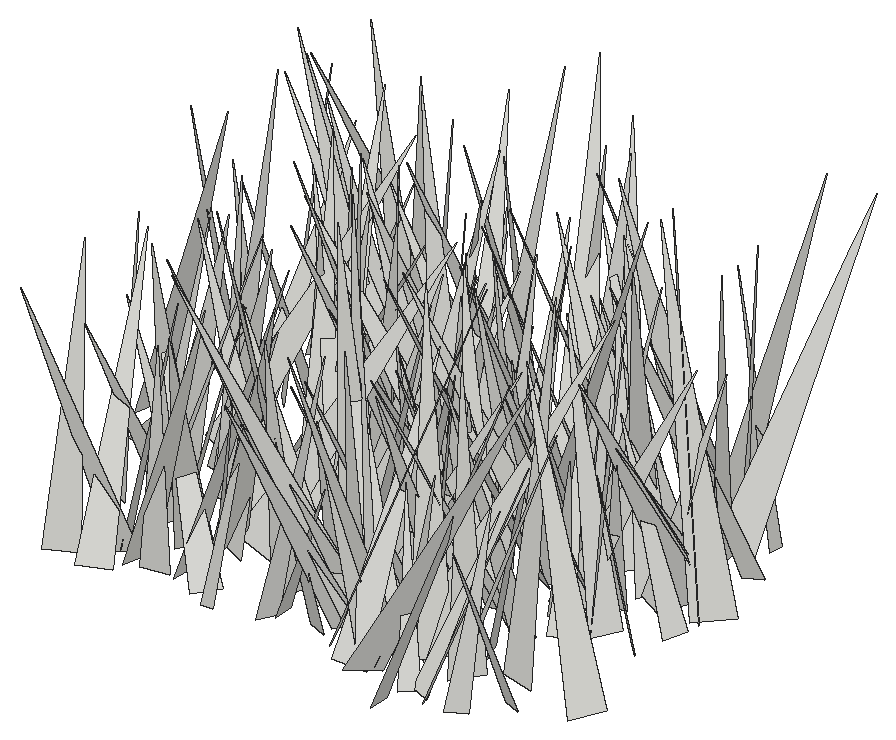
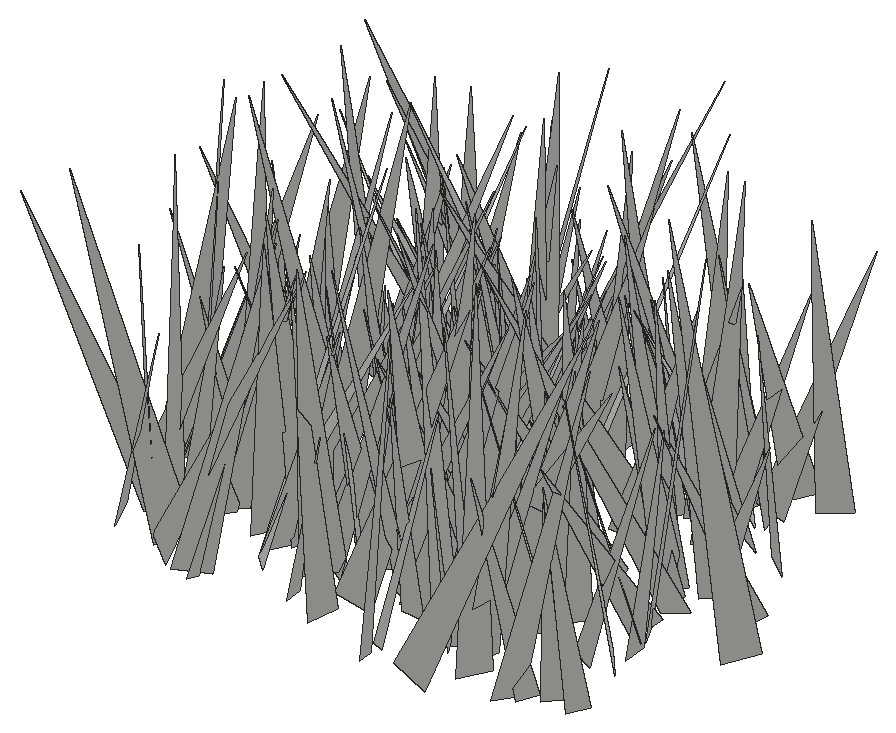
# SketchUp Ruby script. Lengths in inches.
U = 1.inch
M = Sketchup.active_model
def pt(a) = Geom::Point3d.new(a.map { |v| v * U })
def face(e, loops, mat)
  f = e.add_face(loops[0].map { |a| pt(a) })
  loops[1..].each { |l| e.add_face(l.map { |a| pt(a) }).erase! }
  f.material = f.back_material = mat if mat
  f
end
# faces: each face lists its corners as indices into pts; further lists are holes
def faces(e, pts, list, mat = nil) = list.each { |f| face(e, (f[0].is_a?(Array) ? f : [f]).map { |l| l.map { |i| pts[i] } }, mat) }
# xy, xz, yz: faces in a plane at the given z, y or x. An outline is a flat list of corners, or four numbers for a rectangle; further outlines are holes
def ring(l) = l.size == 4 ? [[l[0], l[1]], [l[2], l[1]], [l[2], l[3]], [l[0], l[3]]] : l.each_slice(2).to_a
def flat(e, list, mat, &to3) = list.each { |f| face(e, (f[0].is_a?(Array) ? f : [f]).map { |l| ring(l).map { |u, v| to3.(u, v) } }, mat) }
def xy(e, z, list, mat = nil) = flat(e, list, mat) { |x, y| [x, y, z] }
def xz(e, y, list, mat = nil) = flat(e, list, mat) { |x, z| [x, y, z] }
def yz(e, x, list, mat = nil) = flat(e, list, mat) { |y, z| [x, y, z] }
def lines(e, pts, list) = list.each { |a, b| e.add_line(pt(pts[a]), pt(pts[b])) }
# prism: a flat outline (further loops are holes) pulled along v
def prism(e, loops, v, mat = nil)
  f = face(e, loops, mat); d = Geom::Vector3d.new(v.map { |x| x * U })
  f.pushpull(f.normal.samedirection?(d) ? d.length : -d.length)
end
def box(e, o, s, mat = nil) = prism(e, [[o, [o[0] + s[0], o[1], o[2]], [o[0] + s[0], o[1] + s[1], o[2]], [o[0], o[1] + s[1], o[2]]]], [0, 0, s[2]], mat)
def at(x, y, z, deg = 0) = Geom::Transformation.translation(pt([x, y, z])) * Geom::Transformation.rotation(ORIGIN, Z_AXIS, deg.degrees)
def axes(o, x, y, z) = Geom::Transformation.new([*x, 0, *y, 0, *z, 0, *pt(o).to_a, 1])
def part(name) = M.definitions.add(name)
# library, detail: a bought-in or finely detailed component or shape, given as its bounding box
def library(name, o, s) = part(name).tap { |d| box(d.entities, o, s) }
def detail(e, o, s) = box(e.add_group.entities, o, s)
def put(e, d, t, mat = nil) = e.add_instance(d, t).tap { |i| i.material = mat if mat }
def group(e, t, mat = nil) = e.add_group.tap { |g| g.transformation = t; g.material = mat if mat }.entities
root = M.entities
c1 = part("fur_instance\#9")
p = [[0.8125,0,1.79],[0.67,-0.02,1.48],[0,-0.11,0],[0,0.11,0]]
faces(c1.entities,p,[[0,1,2,3]])
put(root,c1,axes([517.64,24.74,-21.86],[1.43774,-5.64122,0.58152],[-5.34924,-1.54822,-1.79367],[-1.88339,0.09091,5.53834]))
put(root,c1,axes([526.01,23.85,-21.86],[-1.2303,-3.6424,0.32202],[-3.65502,1.23499,0.00478],[0.10759,0.30356,3.84457]))
put(root,c1,axes([524.72,22.25,-21.86],[-2.57998,2.99071,1.64125],[3.02202,2.95835,-0.64026],[1.58287,-0.77341,3.89753]))
put(root,c1,axes([518.1875,25.03,-21.86],[-8.04638,-2.10125,0.20494],[-2.02323,7.90531,1.61682],[0.60315,-1.51404,8.15753]))
put(root,c1,axes([519.22,25.19,-21.86],[-6.19203,-3.31038,1.54754],[-2.85802,6.28451,2.00782],[2.2771,-1.114,6.72819]))
put(root,c1,axes([507.86,24.08,-21.86],[-0.4063,-5.76079,1.26429],[-5.69006,0.04941,-1.60344],[-1.5519,1.32705,5.54804]))
put(root,c1,axes([508.55,24.05,-21.86],[6.83641,-1.96558,0.32372],[-1.94381,-6.83529,-0.45298],[-0.43579,-0.34652,7.09893]))
put(root,c1,axes([509.57,23.6,-21.86],[1.49528,-4.80686,1.53266],[-5.04418,-1.45777,0.34917],[-0.10564,1.56838,5.02194]))
put(root,c1,axes([522.05,21.04,-21.86],[6.47636,2.00005,0.90058],[1.74291,-6.39683,1.67254],[-1.33173,1.35459,6.56857]))
put(root,c1,axes([519.69,23.4375,-21.86],[-4.79801,0.15244,1.14259],[0.25589,4.91001,0.4195],[1.12396,-0.46714,4.78206]))
put(root,c1,axes([520.09,22.57,-21.86],[7.15691,-3.14413,0.26361],[-3.09126,-6.8566,2.14652],[0.63178,2.06831,7.5166]))
put(root,c1,axes([505.98,22.61,-21.86],[3.27303,-4.65782,3.06275],[-5.40234,-3.52629,0.41046],[-1.37496,2.76738,5.67799]))
put(root,c1,axes([522.38,22.42,-21.86],[-3.13044,2.30171,0.23571],[2.28042,3.13636,-0.34054],[0.39127,0.13578,3.8706]))
put(root,c1,axes([515.16,24.08,-21.86],[3.6641,-0.22277,0.06955],[-0.2117,-3.63329,-0.48425],[-0.09821,-0.47926,3.63879]))
put(root,c1,axes([509.48,25.99,-21.86],[4.70982,-4.44224,0.12242],[-4.38661,-4.67586,-0.90827],[-0.71149,-0.57769,6.41023]))
put(root,c1,axes([517.25,26.03,-21.86],[3.98276,-1.20965,1.22676],[-0.42908,-3.68899,-2.24451],[-1.66855,-1.93873,3.5054]))
put(root,c1,axes([522.8125,22.5,-21.86],[0.96645,3.75371,0.08435],[3.72936,-0.9496,-0.47076],[0.43512,-0.19848,3.84744]))
put(root,c1,axes([521.02,23.74,-21.86],[4.01363,-0.60213,1.19124],[-0.70216,-4.16285,0.26162],[-1.13516,0.446,4.0501]))
put(root,c1,axes([518.45,24.46,-21.86],[5.75232,0.0292,2.58276],[0.25276,-6.28131,-0.49192],[-2.57052,-0.55229,5.73133]))
put(root,c1,axes([514.51,25.16,-21.86],[5.42089,-2.3865,1.81758],[-2.19868,-5.71457,-0.94576],[-2.04078,-0.18248,5.84696]))
put(root,c1,axes([520.23,23.57,-21.86],[5.44846,0.74036,0.07595],[0.73692,-5.44519,0.21553],[-0.10422,0.20337,5.4943]))
put(root,c1,axes([523.26,22.27,-21.86],[4.24517,2.47398,0.29086],[2.34061,-4.15824,1.20716],[-0.85248,0.90284,4.76286]))
put(root,c1,axes([516.91,23.9,-21.86],[-5.12266,-6.1706,2.10185],[-6.50165,4.64284,-2.21548],[-0.47189,3.01719,7.70776]))
put(root,c1,axes([514.92,23.48,-21.86],[5.08359,-0.28901,1.82683],[-0.68576,-5.25683,1.07667],[-1.71772,1.24337,4.97667]))
put(root,c1,axes([523.4,24.53,-21.86],[4.8811,-3.48072,2.77846],[-3.79933,-5.40519,-0.09683],[-2.32386,1.52607,5.99426]))
put(root,c1,axes([523.51,23.6,-21.86],[4.74716,3.3592,0.52437],[3.38285,-4.75689,-0.1518],[-0.33985,-0.42721,5.81349]))
put(root,c1,axes([511.97,23.61,-21.86],[-3.53792,4.34861,0.23075],[4.30519,3.44804,1.02808],[-0.65501,-0.82532,5.51093]))
put(root,c1,axes([519.49,22.55,-21.86],[-1.69129,6.09931,0.73665],[6.01995,1.79783,-1.06428],[1.22654,-0.41345,6.23934]))
put(root,c1,axes([516.08,26.26,-21.86],[4.34393,-1.36952,0.92271],[-1.07858,-4.31928,-1.3331],[-1.25046,-1.03195,4.35524]))
put(root,c1,axes([511.19,25.16,-21.86],[3.83115,1.46002,1.29175],[1.69697,-3.89964,-0.62537],[-0.95945,-1.06731,4.05194]))
put(root,c1,axes([507.37,24.68,-21.86],[5.01565,1.80166,1.23073],[1.89818,-5.12441,-0.23415],[-1.07592,-0.64182,5.32428]))
put(root,c1,axes([514.25,27.18,-21.86],[-5.96811,-4.81477,0.42538],[-4.75156,5.96808,0.88657],[0.88638,-0.42578,7.61672]))
put(root,c1,axes([507.65,22.45,-21.86],[-4.47188,4.60163,0.40246],[4.4512,4.44255,-1.33612],[1.23441,0.65071,6.27595]))
put(root,c1,axes([512.72,22.71,-21.86],[2.07794,4.44656,0.23399],[4.16362,-2.03187,1.63715],[-1.57826,0.49406,4.62704]))
put(root,c1,axes([510.54,26.67,-21.86],[6.88515,-2.28469,0.18682],[-2.24647,-6.84269,-0.88939],[-0.45618,-0.78602,7.19959]))
put(root,c1,axes([507.83,27.18,-21.86],[0.74185,-5.118,0.35857],[-5.01336,-0.80012,-1.04825],[-1.09027,0.19676,5.06413]))
put(root,c1,axes([510.47,24.18,-21.86],[6.55283,1.12937,1.12544],[0.97488,-6.60494,0.95181],[-1.26162,0.76214,6.58096]))
put(root,c1,axes([520.47,27.45,-21.86],[1.50349,-5.86365,0.5049],[-5.82358,-1.55753,-0.74685],[-0.85041,0.2992,6.00709]))
put(root,c1,axes([515.95,25.72,-21.86],[-5.32926,2.77314,1.19327],[2.9808,5.21718,1.1879],[0.47858,-1.6143,5.88899]))
put(root,c1,axes([528.59,25.03,-21.86],[-5.76808,3.66085,1.08427],[3.77252,5.76709,0.59739],[0.58783,-1.08949,6.80556]))
put(root,c1,axes([521.47,24.82,-21.86],[-5.69,4.35692,2.08043],[4.49689,5.95288,-0.16772],[1.75752,-1.1258,7.16454]))
put(root,c1,axes([508.03,27.28,-21.86],[4.78165,-4.93816,1.39024],[-4.88475,-4.96331,-0.82896],[-1.56762,0.40313,6.82367]))
put(root,c1,axes([517.77,23.82,-21.86],[6.75975,3.62956,0.52461],[3.54067,-6.74583,1.04905],[-0.95528,0.68056,7.60048]))
put(root,c1,axes([522,28.78,-21.86],[-4.86076,-4.47494,0.06756],[-4.36579,4.76306,1.38194],[0.98465,-0.972,6.46083]))
put(root,c1,axes([519.0625,25.1,-21.86],[-4.60264,5.20733,0.96805],[5.29634,4.53648,0.77902],[0.04773,-1.24166,6.90606]))
put(root,c1,axes([519.39,26.97,-21.86],[-2.08811,-4.65792,0.59921],[-4.45757,1.75934,-1.85749],[-1.47829,1.27435,4.7546]))
put(root,c1,axes([516.67,26.875,-21.86],[-4.81324,5.46383,3.73935],[6.29264,5.21276,0.48307],[2.05886,-3.15867,7.26549]))
put(root,c1,axes([518.51,24.67,-21.86],[1.43872,7.93621,2.15807],[7.82752,-1.99366,2.11323],[-2.52399,-1.65906,7.7838]))
put(root,c1,axes([525.0625,25.375,-21.86],[2.04699,7.14679,2.15899],[7.40344,-2.23185,0.36858],[-0.96272,-1.9673,7.42502]))
put(root,c1,axes([511.01,26.4,-21.86],[1.57919,4.13225,1.33364],[4.34025,-1.54395,-0.35548],[-0.12772,-1.37428,4.40942]))
put(root,c1,axes([519.71,26.97,-21.86],[4.70905,2.28139,1.77217],[2.5251,-4.89691,-0.40574],[-1.40329,-1.15586,5.21682]))
put(root,c1,axes([520.86,24.77,-21.86],[2.72489,7.5123,0.23605],[7.26372,-2.56761,-2.13568],[1.931,-0.94238,7.70056]))
put(root,c1,axes([523.02,28.23,-21.86],[-0.18696,-5.47828,1.21386],[-5.53827,-0.01495,-0.92048],[-0.90141,1.22808,5.40363]))
put(root,c1,axes([508.27,24.54,-21.86],[4.52328,4.39752,0.22155],[4.10164,-4.32376,2.0806],[-1.60118,1.34692,5.95561]))
put(root,c1,axes([515.49,29.15,-21.86],[-3.4189,-2.83051,0.24342],[-2.77437,3.40847,0.66713],[0.61145,-0.36118,4.38812]))
put(root,c1,axes([517.16,28.14,-21.86],[2.82245,-3.27125,1.23973],[-3.47956,-2.78972,0.56063],[-0.36142,1.31172,4.28404]))
put(root,c1,axes([505.17,27.0625,-21.86],[2.73063,4.59292,1.67983],[4.59916,-3.06583,0.90635],[-1.66266,-0.93747,5.2659]))
put(root,c1,axes([522.95,26.5,-21.86],[6.22186,3.72093,2.03459],[3.43335,-6.54009,1.46143],[-2.48938,0.27987,7.10078]))
put(root,c1,axes([519.5,28.74,-21.86],[-3.50463,1.38607,1.3282],[1.66931,3.56562,0.68373],[0.94799,-1.15452,3.70623]))
put(root,c1,axes([507.08,26.35,-21.86],[2.36342,5.34352,0.74133],[5.25737,-2.46286,0.99138],[-1.20944,-0.26392,5.75813]))
put(root,c1,axes([507.03,28.88,-21.86],[4.88196,1.64498,0.71636],[1.77456,-4.73338,-1.22423],[-0.26474,-1.39349,5.00407]))
put(root,c1,axes([520.94,29.14,-21.86],[-1.8038,-4.78632,0.84713],[-4.75617,1.55162,-1.36069],[-1.00264,1.25053,4.93062]))
put(root,c1,axes([523.84,31.3,-21.86],[-2.90473,-5.90083,0.221],[-5.68544,2.86131,1.67173],[1.5951,-0.54696,6.36102]))
put(root,c1,axes([517.11,27.54,-21.86],[2.90433,5.023,0.38727],[4.82562,-2.64532,-1.87916],[1.44702,-1.25991,5.48948]))
put(root,c1,axes([523.43,29.86,-21.86],[0.93641,-4.49496,0.58968],[-4.44892,-0.79539,1.00188],[0.87152,0.76939,4.48082]))
put(root,c1,axes([515.24,28.85,-21.86],[5.83146,1.27805,1.15338],[1.33487,-5.92923,-0.17895],[-1.08712,-0.42484,5.96719]))
put(root,c1,axes([510.91,28.69,-21.86],[-2.86629,5.19134,1.30889],[5.27356,2.48156,1.70596],[-0.92348,-1.94182,5.67938]))
put(root,c1,axes([520.86,31.95,-21.86],[-3.40543,-6.99905,0.02732],[-6.9991,3.40539,-0.01642],[-0.00281,0.03175,7.78353]))
put(root,c1,axes([518.53,30.54,-21.86],[-3.7934,-3.57067,0.95546],[-3.47781,3.9116,0.81037],[1.25196,0.04698,5.14615]))
put(root,c1,axes([511.25,27.2,-21.86],[-0.59602,7.49567,1.64856],[6.68012,1.32078,-3.59019],[3.77872,-1.15261,6.60687]))
put(root,c1,axes([526.86,29.875,-21.86],[-2.53419,-2.69204,0.92744],[-2.77792,2.61003,-0.01451],[0.6248,0.68554,3.69715]))
put(root,c1,axes([507.12,30.71,-21.86],[1.45023,-6.39796,1.08768],[-6.25164,-1.07813,1.99368],[1.74182,1.45734,6.24998]))
put(root,c1,axes([506.11,29.1875,-21.86],[-1.40668,3.30295,0.84871],[3.29754,1.08331,1.24951],[-0.86952,-1.23511,3.36556]))
put(root,c1,axes([521.91,32.16,-21.86],[2.52782,-6.77606,0.30453],[-6.73549,-2.54598,-0.74076],[-0.80053,0.02468,7.19418]))
put(root,c1,axes([505.4,30.24,-21.86],[2.93008,-5.46925,1.49234],[-5.65269,-2.69042,1.23848],[0.43226,1.89052,6.07982]))
put(root,c1,axes([508.35,29.22,-21.86],[1.54209,5.92638,1.72605],[6.04197,-1.81335,0.82809],[-1.2633,-1.43843,6.06748]))
put(root,c1,axes([524.21,28.9375,-21.86],[-1.31854,4.49628,0.43937],[4.51767,1.31381,0.11263],[0.01505,-0.45333,4.68427]))
put(root,c1,axes([506.58,31.32,-21.86],[1.31964,-4.20384,0.49444],[-3.9297,-1.02429,1.77946],[1.57296,0.96785,4.03079]))
put(root,c1,axes([503.22,30.69,-21.86],[2.58418,-3.37784,0.00054],[-2.92311,-2.23595,2.1316],[1.69269,1.29557,3.68023]))
put(root,c1,axes([519.58,30.18,-21.86],[-3.57367,4.96866,1.72232],[5.21894,3.60663,0.42422],[0.64547,-1.65218,6.10563]))
put(root,c1,axes([525.36,30.16,-21.86],[-5.60882,2.54428,1.1021],[2.59069,5.69507,0.03704],[0.9881,-0.48955,6.15881]))
put(root,c1,axes([524.33,31.97,-21.86],[0.84886,-4.32385,0.54485],[-4.30912,-0.7498,0.76315],[0.65118,0.6747,4.3398]))
put(root,c1,axes([524.64,30.01,-21.86],[-3.91577,-3.49387,3.17429],[-4.26524,4.38586,-0.43413],[2.02262,2.48468,5.2299]))
put(root,c1,axes([514.11,30.24,-21.86],[-0.00345,4.9845,1.60202],[5.18158,-0.22632,0.71534],[-0.75028,-1.58596,4.93291]))
put(root,c1,axes([526.41,34.08,-21.86],[4.00993,-5.51552,0.33203],[-5.14979,-3.87921,-2.24547],[-2.00271,-1.06842,6.43882]))
put(root,c1,axes([520.71,32.9375,-21.86],[-6.87561,-0.89332,0.66489],[-0.69538,6.69239,1.80069],[0.86979,-1.71115,6.69549]))
put(root,c1,axes([523.125,30.48,-21.86],[0.63179,6.0642,2.01169],[5.81387,0.29266,-2.70812],[2.6496,-2.08816,5.46258]))
put(root,c1,axes([518.3,31.92,-21.86],[-2.43401,-4.94438,0.27236],[-4.40728,2.02468,-2.63096],[-2.25763,1.37813,4.84245]))
put(root,c1,axes([517.22,32.18,-21.86],[2.03296,-3.43324,0.36978],[-3.45285,-2.01606,0.26469],[0.04074,0.45292,3.9812]))
put(root,c1,axes([522.57,32.8,-21.86],[-1.29347,-4.18784,0.40951],[-4.17089,1.33267,0.45438],[0.55623,0.25449,4.35943]))
put(root,c1,axes([515.72,31.0625,-21.86],[5.7925,1.49056,1.34896],[1.52882,-5.93778,-0.00376],[-1.30544,-0.3399,5.9812]))
put(root,c1,axes([512.96,31.46,-21.86],[-2.66914,2.15187,1.53787],[2.38339,2.90414,0.07299],[1.14676,-1.02728,3.42776]))
put(root,c1,axes([523.29,31.23,-21.86],[-2.34168,-2.41248,1.9117],[-2.76899,2.70012,0.01564],[1.3444,1.35921,3.36204]))
put(root,c1,axes([527.4,31.65,-21.86],[-3.9914,1.89648,0.82188],[2.01712,3.964,0.64912],[0.45094,-0.94526,4.3711]))
put(root,c1,axes([514.66,33.35,-21.86],[-0.7364,-6.55979,0.93298],[-6.36781,0.44127,-1.92351],[-1.83094,1.10364,6.31453]))
put(root,c1,axes([515.47,31.5,-21.86],[-1.82115,-3.36265,1.61921],[-3.73204,1.65736,-0.7556],[0.03439,1.7865,3.74875]))
put(root,c1,axes([512.54,31.41,-21.86],[4.06784,5.47307,2.7985],[5.78633,-4.54195,0.47187],[-2.07475,-1.93641,6.80288]))
put(root,c1,axes([519.1,30.01,-21.86],[-6.05954,0.33778,0.89505],[0.02694,5.79744,-2.00555],[0.95629,1.97708,5.728]))
put(root,c1,axes([501.85,33.27,-21.86],[8.0282,-2.33719,0.44231],[-2.30718,-8.02996,-0.55383],[-0.57877,-0.40914,8.34313]))
put(root,c1,axes([517.36,31.74,-21.86],[-1.86227,-3.58892,1.59018],[-3.91628,1.57852,-1.02377],[-0.26793,1.87217,3.91156]))
put(root,c1,axes([526.7,35.01,-21.86],[-4.06772,-3.26977,0.32403],[-2.78571,3.7053,2.41936],[1.74246,-1.70943,4.62433]))
put(root,c1,axes([511.43,30.99,-21.86],[1.43263,3.39143,0.32506],[3.34277,-1.46736,0.57677],[-0.65831,-0.07043,3.63615]))
put(root,c1,axes([515.86,33.27,-21.86],[4.04014,-3.74392,1.13553],[-3.80741,-4.13804,-0.09691],[-0.90002,0.69913,5.50729]))
put(root,c1,axes([505.65,33.9375,-21.86],[-6.01698,-4.0059,2.23214],[-3.85326,6.41302,1.12219],[2.48637,0.24439,7.14087]))
put(root,c1,axes([519.27,31.54,-21.86],[1.06492,5.99669,1.55027],[6.17359,-1.15473,0.22589],[-0.50038,-1.48458,6.08632]))
put(root,c1,axes([514.15,33.63,-21.86],[-5.99234,-4.15881,0.58341],[-4.19764,5.96205,-0.6148],[0.12593,0.83815,7.26814]))
put(root,c1,axes([511.26,30.85,-21.86],[-5.83364,4.02968,1.05878],[3.90844,5.92385,-1.01134],[1.44341,0.24573,7.01761]))
put(root,c1,axes([512.14,31.56,-21.86],[-5.57386,3.34507,0.61319],[3.34749,5.6042,-0.14346],[0.5998,-0.19191,6.49898]))
put(root,c1,axes([510.21,33.02,-21.86],[5.45486,-2.53583,1.72286],[-2.73109,-5.61705,0.37948],[-1.39279,1.08278,6.00349]))
put(root,c1,axes([518.63,33.77,-21.86],[0.40641,-5.35004,1.66525],[-5.54368,-0.62666,-0.66032],[-0.81458,1.59547,5.32467]))
put(root,c1,axes([507.16,30.78,-21.86],[-7.30658,0.78889,2.52937],[0.00726,7.42557,-2.29501],[2.64953,2.15518,6.98151]))
put(root,c1,axes([518.52,34.28,-21.86],[4.42301,-0.66017,1.25029],[-0.31732,-4.46498,-1.23502],[-1.37781,-1.09094,4.29808]))
put(root,c1,axes([515.54,34.4375,-21.86],[-6.69596,1.51903,0.23584],[1.52209,6.40398,1.96756],[-0.2152,-1.96993,6.57815]))
put(root,c1,axes([515.375,30.52,-21.86],[1.15921,7.66569,0.40932],[7.66684,-1.17697,0.3294],[-0.3873,-0.35503,7.74584]))
put(root,c1,axes([517.72,32.74,-21.86],[2.94995,3.39967,1.09614],[3.50655,-3.02709,-0.04841],[-0.68072,-0.86052,4.50085]))
put(root,c1,axes([508.97,31.46,-21.86],[5.85572,0.96623,0.0245],[0.91904,-5.61274,1.69591],[-0.29926,1.66948,5.68743]))
put(root,c1,axes([512.08,33.45,-21.86],[-0.77614,4.62516,2.62163],[4.88719,1.66369,-1.48826],[2.09294,-2.16967,4.44742]))
put(root,c1,axes([522.83,35.64,-21.86],[0.39282,-7.92697,1.06347],[-7.86049,-0.18606,1.51663],[1.47665,1.11832,7.79044]))
put(root,c1,axes([519.61,33.48,-21.86],[8.28106,0.30024,0.90595],[0.31898,-8.32832,-0.15571],[-0.89952,-0.18935,8.28504]))
put(root,c1,axes([525.25,32.89,-21.86],[2.00403,4.77087,1.2081],[4.88814,-1.77806,-1.08691],[0.57161,-1.52123,5.05925]))
put(root,c1,axes([508.25,34.8,-21.86],[5.02867,-2.50397,0.95955],[-2.41233,-5.11484,-0.70513],[-1.17101,-0.21602,5.57317]))
put(root,c1,axes([520.79,34.5,-21.86],[-2.94744,-5.34651,0.76174],[-5.29498,2.69026,-1.60576],[-1.06233,1.42484,5.89017]))
put(root,c1,axes([527.79,33.42,-21.86],[-4.55755,6.1935,2.40469],[6.62517,4.45559,1.08074],[0.49905,-2.58872,7.61332]))
put(root,c1,axes([527.07,33.33,-21.86],[-5.85102,-5.01294,3.05498],[-5.59861,6.06235,-0.77491],[1.76582,2.61061,7.66574]))
put(root,c1,axes([505.875,32.04,-21.86],[1.59933,7.72158,1.03232],[7.26868,-1.09996,-3.03359],[2.80263,-1.55359,7.2786]))
put(root,c1,axes([512.26,33.94,-21.86],[4.77754,4.17311,2.72058],[4.61145,-5.13068,-0.22808],[-1.8844,-1.97551,6.33938]))
put(root,c1,axes([511.39,31.11,-21.86],[-1.39232,7.88876,0.40308],[7.89477,1.37627,0.33483],[-0.26016,-0.45487,8.00369]))
put(root,c1,axes([510.87,35.13,-21.86],[0.4901,-6.09421,1.40714],[-6.12992,-0.18765,1.32232],[1.24239,1.47818,5.96918]))
put(root,c1,axes([512.84,32.0625,-21.86],[-3.36626,3.2291,1.55087],[2.48228,3.63709,-2.18492],[2.58275,0.71309,4.12128]))
put(root,c1,axes([523.21,31.53,-21.86],[3.09687,5.17866,0.3937],[4.90573,-3.06729,1.75775],[-1.70508,0.58082,5.7723]))
put(root,c1,axes([524.86,33.62,-21.86],[-6.31107,2.62453,1.38258],[2.63294,6.45317,-0.23139],[1.36651,-0.31261,6.83112]))
put(root,c1,axes([514.12,34.75,-21.86],[2.26565,-5.57265,3.25786],[-5.77256,-3.29433,-1.62055],[-2.88887,2.21229,5.79322]))
put(root,c1,axes([505.61,34.46,-21.86],[3.56732,3.05528,0.6125],[3.0981,-3.37772,-1.19517],[0.33415,-1.30074,4.54225]))
put(root,c1,axes([515.41,33.82,-21.86],[-7.4138,3.10521,1.79195],[3.13289,7.61249,-0.22981],[1.74312,-0.47482,8.03455]))
put(root,c1,axes([514.16,32.77,-21.86],[-0.74484,5.04348,0.31723],[4.84937,0.80355,-1.38926],[1.42161,-0.09859,4.90524]))
put(root,c1,axes([513.21,36,-21.86],[2.55159,-4.81811,0.15811],[-4.66384,-2.42197,1.46026],[1.21971,0.81832,5.25284]))
put(root,c1,axes([508.55,36.11,-21.86],[4.04472,-2.80495,1.23292],[-2.68281,-4.22845,-0.81868],[-1.47998,-0.00072,4.85358]))
put(root,c1,axes([522.98,34.34,-21.86],[-3.74669,3.50171,1.17991],[3.59906,3.83892,0.03541],[0.8372,-0.8322,5.12819]))
put(root,c1,axes([521.82,35.27,-21.86],[-5.18196,-4.15409,0.26027],[-4.02731,4.89921,-1.98883],[-1.05116,1.70828,6.3367]))
put(root,c1,axes([517.375,34.98,-21.86],[-5.00491,-0.78513,1.46412],[-0.94309,5.16869,-0.45214],[1.36772,0.69095,5.0459]))
put(root,c1,axes([509.98,33.78,-21.86],[-5.27031,-0.93158,1.82448],[-1.52104,5.15288,-1.7627],[1.37223,2.13373,5.05341]))
put(root,c1,axes([513.37,37.64,-21.86],[3.93068,-5.30389,1.53813],[-4.85639,-4.21869,-2.1367],[-2.62918,-0.13704,6.24628]))
put(root,c1,axes([524.55,37.01,-21.86],[3.93846,-2.19121,0.70559],[-1.95473,-3.92185,-1.26841],[-1.21585,-0.79274,4.32481]))
put(root,c1,axes([505.125,35.38,-21.86],[-4.88413,-0.13594,1.40409],[-0.16648,5.08029,-0.08723],[1.4008,0.12978,4.88524]))
put(root,c1,axes([526.97,36.75,-21.86],[-0.6126,-5.21006,0.97224],[-5.10965,0.32064,-1.50131],[-1.40764,1.1035,5.02654]))
put(root,c1,axes([520.01,38.6,-21.86],[-5.57338,-5.53642,0.81265],[-5.27737,5.58191,1.83481],[1.86058,-0.75178,7.63858]))
put(root,c1,axes([516.1,36.08,-21.86],[-6.12139,2.10353,0.29479],[2.12072,6.0019,1.20952],[-0.1196,-1.23917,6.35872]))
put(root,c1,axes([523.33,36.6,-21.86],[-5.2528,1.04607,1.18822],[1.28573,5.22141,1.0871],[0.92359,-1.31932,5.24446]))
put(root,c1,axes([523.86,36.53,-21.86],[-5.37487,-0.5228,0.79074],[-0.44432,5.41107,0.55741],[0.83736,-0.48456,5.37139]))
put(root,c1,axes([506.35,36.9,-21.86],[-1.82389,-4.57282,0.8897],[-4.65371,1.74485,-0.5721],[-0.21262,1.03617,4.88978]))
put(root,c1,axes([525.46,36.81,-21.86],[6.36794,0.62079,2.33056],[0.97414,-6.68136,-0.88201],[-2.20634,-1.15823,6.33704]))
put(root,c1,axes([515.25,35.03,-21.86],[-4.28711,2.60894,1.39768],[2.40918,4.50508,-1.01958],[1.71929,0.19268,4.91389]))
put(root,c1,axes([511.58,35.66,-21.86],[3.95352,-1.35205,0.74696],[-1.51739,-3.78343,1.18299],[-0.28899,1.3689,4.00736]))
put(root,c1,axes([510.82,39.21,-21.86],[8.12463,-0.31909,0.21051],[-0.21684,-7.53553,-3.0536],[-0.31483,-3.04462,7.53571]))
put(root,c1,axes([515.51,38.85,-21.86],[0.28426,-7.43419,0.75555],[-7.30944,-0.43371,-1.51752],[-1.55247,0.68085,7.28321]))
put(root,c1,axes([517.84,37.22,-21.86],[-3.53449,-6.31522,1.62159],[-6.50822,3.306,-1.31053],[-0.39309,2.04757,7.11738]))
put(root,c1,axes([517.54,35.16,-21.86],[-4.48164,3.41054,1.04148],[3.17852,4.57879,-1.31654],[1.61662,0.45221,5.47573]))
put(root,c1,axes([523.32,36.09,-21.86],[-5.13567,3.95215,0.39173],[3.97037,5.09374,0.66187],[-0.09557,-0.76314,6.44644]))
put(root,c1,axes([516,37.53,-21.86],[4.93042,2.67254,1.54888],[2.99605,-4.84755,-1.1728],[-0.75178,-1.79146,5.48417]))
put(root,c1,axes([510.16,36.62,-21.86],[-2.53782,7.33959,2.16761],[7.45924,1.86167,2.42953],[-1.71111,-2.77006,7.37615]))
put(root,c1,axes([505.88,33.7,-21.86],[-4.95607,3.58078,0.35964],[3.00453,4.45388,-2.94106],[1.98095,2.2034,5.36049]))
put(root,c1,axes([512.18,36.11,-21.86],[-2.8355,7.09509,0.7949],[6.33308,2.10473,3.80453],[-3.2961,-2.05963,6.62616]))
put(root,c1,axes([519.49,36.2,-21.86],[5.828,-3.21448,3.45143],[-4.0564,-6.21538,1.06086],[-2.40642,2.69201,6.57061]))
put(root,c1,axes([514.96,35.12,-21.86],[-3.64093,6.72533,0.73654],[6.73348,3.68347,-0.34805],[0.65778,-0.48058,7.63972]))
put(root,c1,axes([510.49,37.76,-21.86],[-6.63907,0.80935,0.83748],[0.8673,6.67065,0.42894],[0.7773,-0.53025,6.67446]))
put(root,c1,axes([511.59,37.03,-21.86],[-5.60874,-1.91132,2.91151],[-2.48414,6.06379,-0.80475],[2.44113,1.77916,5.87056]))
put(root,c1,axes([520.26,37.39,-21.86],[-5.4054,2.23783,0.44972],[2.26041,5.40869,0.2551],[0.31726,-0.40826,5.84475]))
put(root,c1,axes([505.32,36.36,-21.86],[4.45887,4.52554,1.75159],[4.30275,-4.78695,1.41478],[-2.24387,-0.18639,6.19358]))
put(root,c1,axes([505.92,38.36,-21.86],[4.52674,3.32324,0.78926],[3.39525,-4.2348,-1.64226],[0.37301,-1.78348,5.37013]))
put(root,c1,axes([521.13,36.45,-21.86],[5.10712,-2.96498,5.20518],[-4.57955,-6.3419,0.88079],[-3.86171,3.59957,5.83935]))
put(root,c1,axes([521.27,40.98,-21.86],[-5.21619,-2.22313,1.39253],[-1.54183,5.10575,2.37575],[2.12232,-1.75473,5.14847]))
put(root,c1,axes([513.22,38.21,-21.86],[0.37459,4.6587,1.44665],[4.87681,-0.39143,-0.00226],[-0.11359,-1.44218,4.67373]))
put(root,c1,axes([512.79,40.79,-21.86],[-2.24525,-3.81491,0.32062],[-3.67914,2.25292,1.04201],[1.05843,-0.26136,4.3022]))
put(root,c1,axes([508.73,40.26,-21.86],[7.00851,-2.19777,2.01204],[-2.01969,-7.2848,-0.92211],[-2.19075,-0.31499,7.28692]))
put(root,c1,axes([521.58,40.63,-21.86],[4.80769,-4.80499,2.60276],[-4.52111,-5.44469,-1.70033],[-3.0695,0.49361,6.58109]))
put(root,c1,axes([524.82,38.85,-21.86],[3.82157,4.19761,2.25189],[4.45533,-4.17126,0.21447],[-1.68552,-1.50865,5.67259]))
put(root,c1,axes([509.25,39.21,-21.86],[-7.37907,1.498,2.27835],[1.63074,7.6926,0.22378],[2.18531,-0.6822,7.52626]))
put(root,c1,axes([513.92,37.59,-21.86],[2.95959,7.19025,1.54721],[7.29869,-3.07695,0.338],[-0.90704,-1.29822,7.76818]))
put(root,c1,axes([505.32,39.96,-21.86],[2.68413,-2.59886,0.79499],[-2.66781,-2.73276,0.07385],[-0.51851,0.60713,3.7354]))
put(root,c1,axes([504.12,39.94,-21.86],[3.6262,-2.26105,0.60128],[-2.31235,-3.63241,0.28605],[-0.35624,0.56255,4.26378]))
put(root,c1,axes([523.5,40.13,-21.86],[-4.03956,-5.75099,0.92293],[-5.66396,3.6166,-2.25467],[-1.3584,2.0224,6.65646]))
put(root,c1,axes([506.68,40.86,-21.86],[-6.49711,1.14641,2.18071],[1.63194,6.61021,1.38712],[1.84567,-1.80917,6.45001]))
put(root,c1,axes([510.79,39.1,-21.86],[-3.28983,-1.54802,1.9149],[-2.00034,3.5437,-0.57187],[1.43591,1.38997,3.59058]))
put(root,c1,axes([510.47,41.87,-21.86],[-1.35129,-7.71927,0.81651],[-7.46816,1.06686,-2.27338],[-2.11671,1.16382,7.49966]))
put(root,c1,axes([517.55,39.76,-21.86],[-3.60239,-0.15597,0.87969],[-0.19043,3.7046,-0.12301],[0.87288,0.16452,3.60367]))
put(root,c1,axes([512.67,41.6875,-21.86],[5.99792,1.55177,2.60045],[2.40829,-5.94226,-2.00876],[-1.83589,-2.72525,5.86071]))
put(root,c1,axes([523.83,38.94,-21.86],[7.44072,-1.6859,2.03296],[-2.09272,-7.4711,1.46382],[-1.61112,1.91833,7.48758]))
put(root,c1,axes([525.16,37.85,-21.86],[-0.55252,7.61083,1.2014],[7.43516,0.84266,-1.91879],[2.02152,-1.01911,7.38568]))
put(root,c1,axes([526.23,38.96,-21.86],[-5.16392,-1.1559,0.80889],[-1.35151,4.93357,-1.57791],[0.40477,1.72635,5.05098]))
put(root,c1,axes([517.72,37.81,-21.86],[-5.56313,6.05819,1.00831],[6.02083,5.64819,-0.71719],[1.2116,-0.25113,8.19364]))
put(root,c1,axes([506.125,40.375,-21.86],[3.45367,-2.54495,0.42724],[-2.57712,-3.36456,0.79082],[0.1334,0.88889,4.21654]))
put(root,c1,axes([515.78,40.25,-21.86],[6.28963,-0.96384,2.1084],[-1.07131,-6.61487,0.17192],[-2.05588,0.49827,6.36073]))
